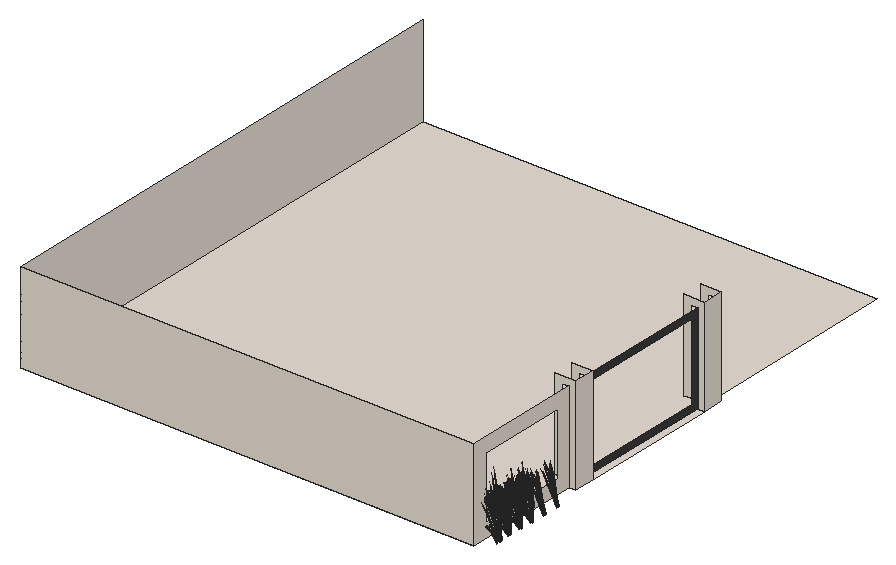
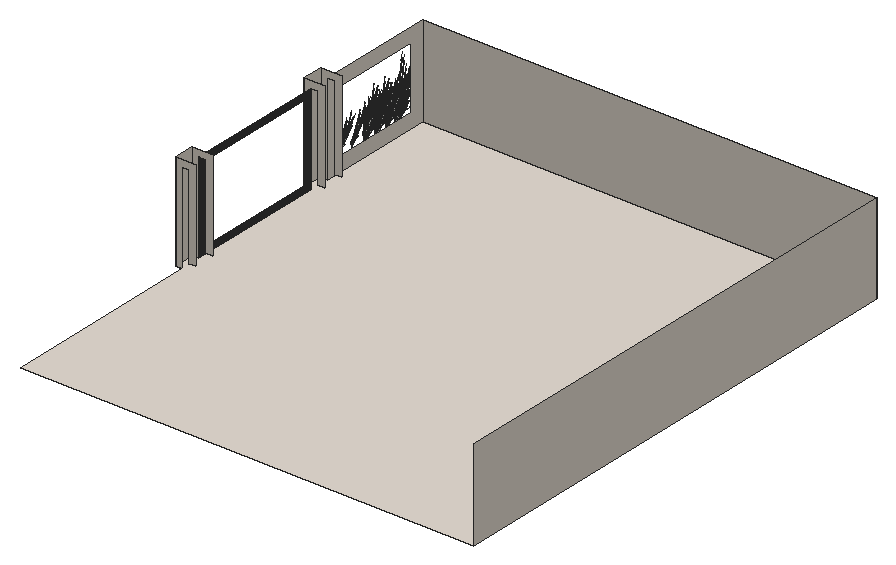
# SketchUp Ruby script. Lengths in inches.
U = 1.inch
M = Sketchup.active_model
def pt(a) = Geom::Point3d.new(a.map { |v| v * U })
def face(e, loops, mat)
  f = e.add_face(loops[0].map { |a| pt(a) })
  loops[1..].each { |l| e.add_face(l.map { |a| pt(a) }).erase! }
  f.material = f.back_material = mat if mat
  f
end
# faces: each face lists its corners as indices into pts; further lists are holes
def faces(e, pts, list, mat = nil) = list.each { |f| face(e, (f[0].is_a?(Array) ? f : [f]).map { |l| l.map { |i| pts[i] } }, mat) }
# xy, xz, yz: faces in a plane at the given z, y or x. An outline is a flat list of corners, or four numbers for a rectangle; further outlines are holes
def ring(l) = l.size == 4 ? [[l[0], l[1]], [l[2], l[1]], [l[2], l[3]], [l[0], l[3]]] : l.each_slice(2).to_a
def flat(e, list, mat, &to3) = list.each { |f| face(e, (f[0].is_a?(Array) ? f : [f]).map { |l| ring(l).map { |u, v| to3.(u, v) } }, mat) }
def xy(e, z, list, mat = nil) = flat(e, list, mat) { |x, y| [x, y, z] }
def xz(e, y, list, mat = nil) = flat(e, list, mat) { |x, z| [x, y, z] }
def yz(e, x, list, mat = nil) = flat(e, list, mat) { |y, z| [x, y, z] }
def lines(e, pts, list) = list.each { |a, b| e.add_line(pt(pts[a]), pt(pts[b])) }
# prism: a flat outline (further loops are holes) pulled along v
def prism(e, loops, v, mat = nil)
  f = face(e, loops, mat); d = Geom::Vector3d.new(v.map { |x| x * U })
  f.pushpull(f.normal.samedirection?(d) ? d.length : -d.length)
end
def box(e, o, s, mat = nil) = prism(e, [[o, [o[0] + s[0], o[1], o[2]], [o[0] + s[0], o[1] + s[1], o[2]], [o[0], o[1] + s[1], o[2]]]], [0, 0, s[2]], mat)
def at(x, y, z, deg = 0) = Geom::Transformation.translation(pt([x, y, z])) * Geom::Transformation.rotation(ORIGIN, Z_AXIS, deg.degrees)
def axes(o, x, y, z) = Geom::Transformation.new([*x, 0, *y, 0, *z, 0, *pt(o).to_a, 1])
def part(name) = M.definitions.add(name)
# library, detail: a bought-in or finely detailed component or shape, given as its bounding box
def library(name, o, s) = part(name).tap { |d| box(d.entities, o, s) }
def detail(e, o, s) = box(e.add_group.entities, o, s)
def put(e, d, t, mat = nil) = e.add_instance(d, t).tap { |i| i.material = mat if mat }
def group(e, t, mat = nil) = e.add_group.tap { |g| g.transformation = t; g.material = mat if mat }.entities
root = M.entities
M.materials.add("LightPink_Translucent").color = [144, 107, 117]
M.materials["LightPink_Translucent"].alpha = 0.75
M.materials.add("M07_Charcoal_Gleam").color = [58, 58, 58]
M.materials.add("Marble_01_1K").color = [230, 221, 211]
c1 = part("blade")
p = [[2.15,0.21,22],[0,0.17,0],[0.09,0.45,0],[2.18,0.31,22],[2.29,0.31,22],[0.38,0.45,0],
  [2.48,0.24,33],[2.49,0.24,33],[2.48,0.22,33]]
faces(c1.entities,p,[[0,1,2,3],[4,5,2,3],[6,3,4,7],[8,0,3,6]])
c2 = part("seeds")
p = [[0.3,-0.1,1.38],[-0.01,-0.03,1.59],[-0.01,-0.03,0.03],[0.14,-0.07,-0.07],[0.29,-0.03,3],[0.15,0.01,3.11]]
faces(c2.entities,p,[[0,1,2,3],[1,0,4,5]],"LightPink_Translucent")
c3 = part("blade with seeds")
put(c3.entities,c1,at(0,0,0))
put(c3.entities,c2,axes([2.4,0.25,30.99],[1.5799,-0.05474,1.17369],[-0.12525,1.92788,0.29478],[-0.07173,-0.02425,1.56792]))
xy(root,-12,[[0,0,0,432,390,432,390,258,396,258,396,240,390,240,390,120,396,120,396,102,390,102,390,0],[390,120,396,240]],"Marble_01_1K")
xz(root,0,[[0,-12,390,66]],"Marble_01_1K")
xz(root,102,[[390,-12,396,-12,396,72,378,72,378,-6,384,-6,384,66,390,66]],"Marble_01_1K")
xz(root,120,[[390,-12,390,66,384,66,384,-6,378,-6,378,72,396,72,396,-12]],"Marble_01_1K")
xz(root,240,[[390,-12,396,-12,396,72,378,72,378,-6,384,-6,384,66,390,66]],"Marble_01_1K")
xz(root,258,[[390,-12,390,66,384,66,384,-6,378,-6,378,72,396,72,396,-12]],"Marble_01_1K")
yz(root,0,[[0,-12,432,66]],"Marble_01_1K")
yz(root,390,[[[120,-12,240,66],[126,-6,234,60]]],"M07_Charcoal_Gleam")
yz(root,390,[[[0,-12,102,66],[12,0,90,54]]],"Marble_01_1K")
yz(root,396,[[102,-12,120,72],[240,-12,258,72]],"Marble_01_1K")
put(root,c3,axes([401.01,11.33,-8.39],[0.21212,-0.01231,1.59586],[-0.14072,0.53355,0.12904],[-0.3023,-0.033,0.68222]))
put(root,c3,axes([401.25,33.91,-8.39],[0.21212,-0.01231,1.59586],[-0.14072,0.53355,0.12904],[-0.3023,-0.033,0.68222]))
put(root,c3,axes([401.28,45.77,-8.39],[0.21212,-0.01231,1.59586],[-0.14072,0.53355,0.12904],[-0.3023,-0.033,0.68222]))
put(root,c3,axes([401.1,12.27,-8.39],[0.17745,-0.11497,1.59586],[0.14939,0.53127,0.12904],[-0.27857,0.12007,0.68222]))
put(root,c3,axes([401.63,21.93,-8.39],[0.21212,-0.01231,1.59586],[-0.14072,0.53355,0.12904],[-0.3023,-0.033,0.68222]))
put(root,c3,axes([400.55,13.17,-9.59],[0.17773,0.04462,1.33163],[0.11455,0.45576,-0.28638],[-0.24142,0.08531,0.56934]))
put(root,c3,axes([401.34,34.85,-8.39],[0.17745,-0.11497,1.59586],[0.14939,0.53127,0.12904],[-0.27857,0.12007,0.68222]))
put(root,c3,axes([401.36,46.71,-8.39],[0.17745,-0.11497,1.59586],[0.14939,0.53127,0.12904],[-0.27857,0.12007,0.68222]))
put(root,c3,axes([402.12,11.71,-8.89],[0.14537,-0.07863,1.64882],[0.05013,0.549,0.12904],[-0.31487,0.07285,0.5893]))
put(root,c3,axes([400.79,35.76,-9.59],[0.17773,0.04462,1.33163],[0.11455,0.45576,-0.28638],[-0.24142,0.08531,0.56934]))
put(root,c3,axes([400.8125,47.62,-9.59],[0.17773,0.04462,1.33163],[0.11455,0.45576,-0.28638],[-0.24142,0.08531,0.56934]))
put(root,c3,axes([402.36,34.3,-8.89],[0.14537,-0.07863,1.64882],[0.05013,0.549,0.12904],[-0.31487,0.07285,0.5893]))
put(root,c3,axes([402.38,46.16,-8.89],[0.14537,-0.07863,1.64882],[0.05013,0.549,0.12904],[-0.31487,0.07285,0.5893]))
put(root,c3,axes([401.72,22.87,-8.39],[0.17745,-0.11497,1.59586],[0.14939,0.53127,0.12904],[-0.27857,0.12007,0.68222]))
put(root,c3,axes([400.56,12.08,-7.61],[-0.08351,0.07057,1.62908],[0.0071,0.51561,-0.25764],[-0.19143,0.06705,0.13065]))
put(root,c3,axes([401.65,10.83,-7.36],[-0.51122,-0.01309,-0.66157],[0.03434,-0.5511,0.07984],[-0.21658,-0.05816,0.93586]))
put(root,c3,axes([401.23,10.97,-9.59],[0.09985,0.15133,1.33163],[-0.23008,0.41134,-0.28638],[-0.23625,-0.09832,0.56934]))
put(root,c3,axes([401.16,23.77,-9.59],[0.17773,0.04462,1.33163],[0.11455,0.45576,-0.28638],[-0.24142,0.08531,0.56934]))
put(root,c3,axes([400.82,11.79,-7.78],[-0.42502,-0.15163,-0.32977],[0.12396,-0.44238,0.42575],[-0.17112,0.04056,0.81462]))
put(root,c3,axes([401.41,10.47,-8.39],[0.18996,0.09365,1.59586],[-0.39312,0.39287,0.12904],[-0.24502,-0.17723,0.68222]))
put(root,c3,axes([400.8,34.67,-7.61],[-0.08351,0.07057,1.62908],[0.0071,0.51561,-0.25764],[-0.19143,0.06705,0.13065]))
put(root,c3,axes([400.82,46.52,-7.61],[-0.08351,0.07057,1.62908],[0.0071,0.51561,-0.25764],[-0.19143,0.06705,0.13065]))
put(root,c3,axes([401.89,33.42,-7.36],[-0.51122,-0.01309,-0.66157],[0.03434,-0.5511,0.07984],[-0.21658,-0.05816,0.93586]))
put(root,c3,axes([402.74,22.3125,-8.89],[0.14537,-0.07863,1.64882],[0.05013,0.549,0.12904],[-0.31487,0.07285,0.5893]))
put(root,c3,axes([401.91,45.28,-7.36],[-0.51122,-0.01309,-0.66157],[0.03434,-0.5511,0.07984],[-0.21658,-0.05816,0.93586]))
put(root,c3,axes([401.48,33.55,-9.59],[0.09985,0.15133,1.33163],[-0.23008,0.41134,-0.28638],[-0.23625,-0.09832,0.56934]))
put(root,c3,axes([401.5,45.41,-9.59],[0.09985,0.15133,1.33163],[-0.23008,0.41134,-0.28638],[-0.23625,-0.09832,0.56934]))
put(root,c3,axes([399.63,12.6,-7.62],[0.06527,0.01458,1.65179],[0.20191,0.48025,-0.15608],[-0.1336,0.12605,0.29231]))
put(root,c3,axes([401.12,12.01,-7.64],[-0.13855,0.49442,-0.47583],[-0.47502,-0.16947,-0.36857],[-0.19125,0.04534,0.91046]))
put(root,c3,axes([401.07,34.37,-7.78],[-0.42502,-0.15163,-0.32977],[0.12396,-0.44238,0.42575],[-0.17112,0.04056,0.81462]))
put(root,c3,axes([401.09,46.23,-7.78],[-0.42502,-0.15163,-0.32977],[0.12396,-0.44238,0.42575],[-0.17112,0.04056,0.81462]))
put(root,c3,axes([401.66,33.06,-8.39],[0.18996,0.09365,1.59586],[-0.39312,0.39287,0.12904],[-0.24502,-0.17723,0.68222]))
put(root,c3,axes([401.68,44.92,-8.39],[0.18996,0.09365,1.59586],[-0.39312,0.39287,0.12904],[-0.24502,-0.17723,0.68222]))
put(root,c3,axes([401.48,10.94,-7.64],[-0.37135,0.36005,-0.47583],[-0.32522,-0.38035,-0.36857],[-0.18868,-0.05478,0.91046]))
put(root,c3,axes([400.875,11.98,-10.61],[0.01297,0.08566,1.6421],[-0.26146,0.44735,-0.25086],[-0.18572,-0.02255,0.2797]))
put(root,c3,axes([399.87,35.1875,-7.62],[0.06527,0.01458,1.65179],[0.20191,0.48025,-0.15608],[-0.1336,0.12605,0.29231]))
put(root,c3,axes([401.17,22.68,-7.61],[-0.08351,0.07057,1.62908],[0.0071,0.51561,-0.25764],[-0.19143,0.06705,0.13065]))
put(root,c3,axes([401.36,34.6,-7.64],[-0.13855,0.49442,-0.47583],[-0.47502,-0.16947,-0.36857],[-0.19125,0.04534,0.91046]))
put(root,c3,axes([399.89,47.05,-7.62],[0.06527,0.01458,1.65179],[0.20191,0.48025,-0.15608],[-0.1336,0.12605,0.29231]))
put(root,c3,axes([402.26,21.43,-7.36],[-0.51122,-0.01309,-0.66157],[0.03434,-0.5511,0.07984],[-0.21658,-0.05816,0.93586]))
put(root,c3,axes([400.95,9.93,-7.62],[0.03791,0.05424,1.65179],[-0.18278,0.48761,-0.15608],[-0.18511,0.00353,0.29231]))
put(root,c3,axes([401.38,46.46,-7.64],[-0.13855,0.49442,-0.47583],[-0.47502,-0.16947,-0.36857],[-0.19125,0.04534,0.91046]))
put(root,c3,axes([401.85,21.56,-9.59],[0.09985,0.15133,1.33163],[-0.23008,0.41134,-0.28638],[-0.23625,-0.09832,0.56934]))
put(root,c3,axes([401.72,33.53,-7.64],[-0.37135,0.36005,-0.47583],[-0.32522,-0.38035,-0.36857],[-0.18868,-0.05478,0.91046]))
put(root,c3,axes([400.18,14.13,-9.42],[0.21313,-0.24635,1.06958],[0.0841,0.38999,0.78586],[-0.15402,0.06983,0.23558]))
put(root,c3,axes([401.74,45.39,-7.64],[-0.37135,0.36005,-0.47583],[-0.32522,-0.38035,-0.36857],[-0.18868,-0.05478,0.91046]))
put(root,c3,axes([401.12,34.57,-10.61],[0.01297,0.08566,1.6421],[-0.26146,0.44735,-0.25086],[-0.18572,-0.02255,0.2797]))
put(root,c3,axes([401.14,46.42,-10.61],[0.01297,0.08566,1.6421],[-0.26146,0.44735,-0.25086],[-0.18572,-0.02255,0.2797]))
put(root,c3,axes([401.44,22.38,-7.78],[-0.42502,-0.15163,-0.32977],[0.12396,-0.44238,0.42575],[-0.17112,0.04056,0.81462]))
put(root,c3,axes([401.375,9.61,-7.61],[-0.11004,-0.00384,1.62908],[-0.35032,0.38367,-0.25764],[-0.18692,-0.07839,0.13065]))
put(root,c3,axes([402.03,21.07,-8.39],[0.18996,0.09365,1.59586],[-0.39312,0.39287,0.12904],[-0.24502,-0.17723,0.68222]))
put(root,c3,axes([400.92,11.73,-7.59],[0.14449,-0.4956,0.447],[0.47502,0.16947,0.36857],[-0.1868,0.02978,0.92496]))
put(root,c3,axes([401.19,32.52,-7.62],[0.03791,0.05424,1.65179],[-0.18278,0.48761,-0.15608],[-0.18511,0.00353,0.29231]))
put(root,c3,axes([401.22,44.38,-7.62],[0.03791,0.05424,1.65179],[-0.18278,0.48761,-0.15608],[-0.18511,0.00353,0.29231]))
put(root,c3,axes([401.09,11.59,-7.3125],[0.25732,0.49218,-0.11324],[-0.45669,0.24187,-0.62851],[-0.19245,0.06494,0.95501]))
put(root,c3,axes([401.67,10.57,-7.3125],[-0.02738,0.55277,-0.11324],[-0.51847,-0.01511,-0.62851],[-0.19968,-0.0384,0.95501]))
put(root,c3,axes([401.34,10.61,-7.78],[-0.29098,-0.34031,-0.32977],[0.33226,-0.32215,0.42575],[-0.16881,-0.04902,0.81462]))
put(root,c3,axes([400.89,11.6,-7.6],[-0.18783,-0.37061,0.05988],[0.34252,-0.1814,0.47138],[-0.15099,0.03579,0.71878]))
put(root,c3,axes([400.42,36.71,-9.42],[0.21313,-0.24635,1.06958],[0.0841,0.38999,0.78586],[-0.15402,0.06983,0.23558]))
put(root,c3,axes([400.25,23.2,-7.62],[0.06527,0.01458,1.65179],[0.20191,0.48025,-0.15608],[-0.1336,0.12605,0.29231]))
put(root,c3,axes([401.73,22.61,-7.64],[-0.13855,0.49442,-0.47583],[-0.47502,-0.16947,-0.36857],[-0.19125,0.04534,0.91046]))
put(root,c3,axes([400.44,48.57,-9.42],[0.21313,-0.24635,1.06958],[0.0841,0.38999,0.78586],[-0.15402,0.06983,0.23558]))
put(root,c3,axes([401.75,12.625,-8.39],[0.12773,-0.16701,1.59586],[0.32252,0.4508,0.12904],[-0.22121,0.20529,0.68222]))
put(root,c3,axes([401.62,32.19,-7.61],[-0.11004,-0.00384,1.62908],[-0.35032,0.38367,-0.25764],[-0.18692,-0.07839,0.13065]))
put(root,c3,axes([400.98,13.0625,-7.78],[-0.44516,0.07768,-0.32977],[-0.11755,-0.44407,0.42575],[-0.12757,0.11927,0.81462]))
put(root,c3,axes([401.64,44.05,-7.61],[-0.11004,-0.00384,1.62908],[-0.35032,0.38367,-0.25764],[-0.18692,-0.07839,0.13065]))
put(root,c3,axes([402.09,21.54,-7.64],[-0.37135,0.36005,-0.47583],[-0.32522,-0.38035,-0.36857],[-0.18868,-0.05478,0.91046]))
put(root,c3,axes([401.17,34.32,-7.59],[0.14449,-0.4956,0.447],[0.47502,0.16947,0.36857],[-0.1868,0.02978,0.92496]))
put(root,c3,axes([401.5,22.58,-10.61],[0.01297,0.08566,1.6421],[-0.26146,0.44735,-0.25086],[-0.18572,-0.02255,0.2797]))
put(root,c3,axes([400.74,14.38,-10.61],[0.0686,0.0543,1.6421],[0.11632,0.50315,-0.25086],[-0.15204,0.10729,0.2797]))
put(root,c3,axes([401.1875,46.17,-7.59],[0.14449,-0.4956,0.447],[0.47502,0.16947,0.36857],[-0.1868,0.02978,0.92496]))
put(root,c3,axes([401.34,34.17,-7.3125],[0.25732,0.49218,-0.11324],[-0.45669,0.24187,-0.62851],[-0.19245,0.06494,0.95501]))
put(root,c3,axes([403.33,72.08,-8.39],[0.21212,-0.01231,1.59586],[-0.14072,0.53355,0.12904],[-0.3023,-0.033,0.68222]))
put(root,c3,axes([403.34,57.84,-8.39],[0.21212,-0.01231,1.59586],[-0.14072,0.53355,0.12904],[-0.3023,-0.033,0.68222]))
put(root,c3,axes([400.64,11.42,-9.42],[0.3265,-0.03889,1.06958],[-0.20711,0.3427,0.78586],[-0.16135,-0.05141,0.23558]))
put(root,c3,axes([401.36,46.03,-7.3125],[0.25732,0.49218,-0.11324],[-0.45669,0.24187,-0.62851],[-0.19245,0.06494,0.95501]))
put(root,c3,axes([401.91,33.15,-7.3125],[-0.02738,0.55277,-0.11324],[-0.51847,-0.01511,-0.62851],[-0.19968,-0.0384,0.95501]))
put(root,c3,axes([401.58,33.19,-7.78],[-0.29098,-0.34031,-0.32977],[0.33226,-0.32215,0.42575],[-0.16881,-0.04902,0.81462]))
put(root,c3,axes([401.9375,45.01,-7.3125],[-0.02738,0.55277,-0.11324],[-0.51847,-0.01511,-0.62851],[-0.19968,-0.0384,0.95501]))
put(root,c3,axes([401.6,45.05,-7.78],[-0.29098,-0.34031,-0.32977],[0.33226,-0.32215,0.42575],[-0.16881,-0.04902,0.81462]))
put(root,c3,axes([401.13,34.18,-7.6],[-0.18783,-0.37061,0.05988],[0.34252,-0.1814,0.47138],[-0.15099,0.03579,0.71878]))
put(root,c3,axes([401.15,46.04,-7.6],[-0.18783,-0.37061,0.05988],[0.34252,-0.1814,0.47138],[-0.15099,0.03579,0.71878]))
put(root,c3,axes([401.57,20.53,-7.62],[0.03791,0.05424,1.65179],[-0.18278,0.48761,-0.15608],[-0.18511,0.00353,0.29231]))
put(root,c3,axes([401.99,35.21,-8.39],[0.12773,-0.16701,1.59586],[0.32252,0.4508,0.12904],[-0.22121,0.20529,0.68222]))
put(root,c3,axes([401.22,35.65,-7.78],[-0.44516,0.07768,-0.32977],[-0.11755,-0.44407,0.42575],[-0.12757,0.11927,0.81462]))
put(root,c3,axes([402.01,47.07,-8.39],[0.12773,-0.16701,1.59586],[0.32252,0.4508,0.12904],[-0.22121,0.20529,0.68222]))
put(root,c3,axes([401.25,47.51,-7.78],[-0.44516,0.07768,-0.32977],[-0.11755,-0.44407,0.42575],[-0.12757,0.11927,0.81462]))
put(root,c3,axes([401.04,12.97,-7.59],[-0.12683,-0.50025,0.447],[0.49754,-0.08682,0.36857],[-0.14663,0.11765,0.92496]))
put(root,c3,axes([400.79,24.73,-9.42],[0.21313,-0.24635,1.06958],[0.0841,0.38999,0.78586],[-0.15402,0.06983,0.23558]))
put(root,c3,axes([400.98,36.97,-10.61],[0.0686,0.0543,1.6421],[0.11632,0.50315,-0.25086],[-0.15204,0.10729,0.2797]))
put(root,c3,axes([401,48.82,-10.61],[0.0686,0.0543,1.6421],[0.11632,0.50315,-0.25086],[-0.15204,0.10729,0.2797]))
put(root,c3,axes([401.99,20.21,-7.61],[-0.11004,-0.00384,1.62908],[-0.35032,0.38367,-0.25764],[-0.18692,-0.07839,0.13065]))
put(root,c3,axes([400.88,34.01,-9.42],[0.3265,-0.03889,1.06958],[-0.20711,0.3427,0.78586],[-0.16135,-0.05141,0.23558]))
put(root,c3,axes([401.29,10.48,-7.26],[0.42234,-0.40113,0.50064],[0.36424,0.42599,0.4128],[-0.19815,-0.07399,1.03595]))
put(root,c3,axes([400.9,45.86,-9.42],[0.3265,-0.03889,1.06958],[-0.20711,0.3427,0.78586],[-0.16135,-0.05141,0.23558]))
put(root,c3,axes([400.9375,12.87,-7.6],[-0.35109,-0.22859,0.05988],[0.2044,-0.32553,0.47138],[-0.11256,0.10524,0.71878]))
put(root,c3,axes([401.54,22.33,-7.59],[0.14449,-0.4956,0.447],[0.47502,0.16947,0.36857],[-0.1868,0.02978,0.92496]))
put(root,c3,axes([401.71,22.1875,-7.3125],[0.25732,0.49218,-0.11324],[-0.45669,0.24187,-0.62851],[-0.19245,0.06494,0.95501]))
put(root,c3,axes([402.29,21.16,-7.3125],[-0.02738,0.55277,-0.11324],[-0.51847,-0.01511,-0.62851],[-0.19968,-0.0384,0.95501]))
put(root,c3,axes([401.28,35.55,-7.59],[-0.12683,-0.50025,0.447],[0.49754,-0.08682,0.36857],[-0.14663,0.11765,0.92496]))
put(root,c3,axes([401.96,21.2,-7.78],[-0.29098,-0.34031,-0.32977],[0.33226,-0.32215,0.42575],[-0.16881,-0.04902,0.81462]))
put(root,c3,axes([401.3,47.41,-7.59],[-0.12683,-0.50025,0.447],[0.49754,-0.08682,0.36857],[-0.14663,0.11765,0.92496]))
put(root,c3,axes([401.51,22.2,-7.6],[-0.18783,-0.37061,0.05988],[0.34252,-0.1814,0.47138],[-0.15099,0.03579,0.71878]))
put(root,c3,axes([401.65,13.04,-8.39],[0.09522,-0.18683,1.59586],[0.39947,0.38663,0.12904],[-0.18021,0.24097,0.68222]))
put(root,c3,axes([402.37,23.22,-8.39],[0.12773,-0.16701,1.59586],[0.32252,0.4508,0.12904],[-0.22121,0.20529,0.68222]))
put(root,c3,axes([401.6,23.66,-7.78],[-0.44516,0.07768,-0.32977],[-0.11755,-0.44407,0.42575],[-0.12757,0.11927,0.81462]))
put(root,c3,axes([401.54,33.0625,-7.26],[0.42234,-0.40113,0.50064],[0.36424,0.42599,0.4128],[-0.19815,-0.07399,1.03595]))
put(root,c3,axes([401.56,44.92,-7.26],[0.42234,-0.40113,0.50064],[0.36424,0.42599,0.4128],[-0.19815,-0.07399,1.03595]))
put(root,c3,axes([403.42,73.02,-8.39],[0.17745,-0.11497,1.59586],[0.14939,0.53127,0.12904],[-0.27857,0.12007,0.68222]))
put(root,c3,axes([403.43,58.78,-8.39],[0.17745,-0.11497,1.59586],[0.14939,0.53127,0.12904],[-0.27857,0.12007,0.68222]))
put(root,c3,axes([401.18,35.45,-7.6],[-0.35109,-0.22859,0.05988],[0.2044,-0.32553,0.47138],[-0.11256,0.10524,0.71878]))
put(root,c3,axes([401.2,47.3125,-7.6],[-0.35109,-0.22859,0.05988],[0.2044,-0.32553,0.47138],[-0.11256,0.10524,0.71878]))
put(root,c3,axes([401.36,24.98,-10.61],[0.0686,0.0543,1.6421],[0.11632,0.50315,-0.25086],[-0.15204,0.10729,0.2797]))
put(root,c3,axes([401.27,11.74,-7.3],[0.42502,0.15163,0.32977],[-0.12396,0.44238,-0.42575],[-0.17112,0.04056,0.81462]))
put(root,c3,axes([401.26,22.02,-9.42],[0.3265,-0.03889,1.06958],[-0.20711,0.3427,0.78586],[-0.16135,-0.05141,0.23558]))
put(root,c3,axes([402.87,73.93,-9.59],[0.17773,0.04462,1.33163],[0.11455,0.45576,-0.28638],[-0.24142,0.08531,0.56934]))
put(root,c3,axes([402.875,59.69,-9.59],[0.17773,0.04462,1.33163],[0.11455,0.45576,-0.28638],[-0.24142,0.08531,0.56934]))
put(root,c3,axes([401.35,13.11,-7.64],[0.13138,0.49631,-0.47583],[-0.49754,0.08682,-0.36857],[-0.14258,0.13331,0.91046]))
put(root,c3,axes([401.9,35.62,-8.39],[0.09522,-0.18683,1.59586],[0.39947,0.38663,0.12904],[-0.18021,0.24097,0.68222]))
put(root,c3,axes([401.92,47.48,-8.39],[0.09522,-0.18683,1.59586],[0.39947,0.38663,0.12904],[-0.18021,0.24097,0.68222]))
put(root,c3,axes([401.49,10.47,-7.6],[0.02575,-0.41332,0.05988],[0.38885,0.01133,0.47138],[-0.14895,-0.04325,0.71878]))
put(root,c3,axes([400.57,14.01,-7.61],[-0.01271,0.10756,1.62908],[0.36076,0.37419,-0.25764],[-0.09444,0.17695,0.13065]))
put(root,c3,axes([401.66,23.5625,-7.59],[-0.12683,-0.50025,0.447],[0.49754,-0.08682,0.36857],[-0.14663,0.11765,0.92496]))
put(root,c3,axes([404.44,72.47,-8.89],[0.14537,-0.07863,1.64882],[0.05013,0.549,0.12904],[-0.31487,0.07285,0.5893]))
put(root,c3,axes([404.45,58.23,-8.89],[0.14537,-0.07863,1.64882],[0.05013,0.549,0.12904],[-0.31487,0.07285,0.5893]))
put(root,c3,axes([402.59,12.76,-10.08],[-0.53199,-0.08911,-0.58063],[0.11226,-0.54969,-0.15239],[-0.15876,-0.06661,1.28164]))
put(root,c3,axes([402.68,9.76,-6.94],[-0.34131,0.52108,-0.12682],[-0.49429,-0.3002,-0.70393],[-0.17182,-0.14722,1.06961]))
put(root,c3,axes([401.52,34.32,-7.3],[0.42502,0.15163,0.32977],[-0.12396,0.44238,-0.42575],[-0.17112,0.04056,0.81462]))
put(root,c3,axes([401.91,21.08,-7.26],[0.42234,-0.40113,0.50064],[0.36424,0.42599,0.4128],[-0.19815,-0.07399,1.03595]))
put(root,c3,axes([401.54,46.18,-7.3],[0.42502,0.15163,0.32977],[-0.12396,0.44238,-0.42575],[-0.17112,0.04056,0.81462]))
put(root,c3,axes([401.75,10.78,-7.3],[0.29098,0.34031,0.32977],[-0.33226,0.32215,-0.42575],[-0.16881,-0.04902,0.81462]))
put(root,c3,axes([401.56,23.47,-7.6],[-0.35109,-0.22859,0.05988],[0.2044,-0.32553,0.47138],[-0.11256,0.10524,0.71878]))
put(root,c3,axes([401.59,35.7,-7.64],[0.13138,0.49631,-0.47583],[-0.49754,0.08682,-0.36857],[-0.14258,0.13331,0.91046]))
put(root,c3,axes([402.53,10.18,-7.36],[-0.43608,-0.26272,-0.66157],[0.30991,-0.46038,0.07984],[-0.158,-0.15687,0.93586]))
put(root,c3,axes([401.61,47.56,-7.64],[0.13138,0.49631,-0.47583],[-0.49754,0.08682,-0.36857],[-0.14258,0.13331,0.91046]))
put(root,c3,axes([402.33,10.2,-7.64],[-0.50465,0.12921,-0.47583],[-0.08828,-0.48932,-0.36857],[-0.13555,-0.14022,0.91046]))
put(root,c3,axes([401.73,33.06,-7.6],[0.02575,-0.41332,0.05988],[0.38885,0.01133,0.47138],[-0.14895,-0.04325,0.71878]))
put(root,c3,axes([400.8125,36.59,-7.61],[-0.01271,0.10756,1.62908],[0.36076,0.37419,-0.25764],[-0.09444,0.17695,0.13065]))
put(root,c3,axes([401.75,44.92,-7.6],[0.02575,-0.41332,0.05988],[0.38885,0.01133,0.47138],[-0.14895,-0.04325,0.71878]))
put(root,c3,axes([400.84,48.45,-7.61],[-0.01271,0.10756,1.62908],[0.36076,0.37419,-0.25764],[-0.09444,0.17695,0.13065]))
put(root,c3,axes([402.83,35.34,-10.08],[-0.53199,-0.08911,-0.58063],[0.11226,-0.54969,-0.15239],[-0.15876,-0.06661,1.28164]))
put(root,c3,axes([402.93,32.34,-6.94],[-0.34131,0.52108,-0.12682],[-0.49429,-0.3002,-0.70393],[-0.17182,-0.14722,1.06961]))
put(root,c3,axes([402.27,23.63,-8.39],[0.09522,-0.18683,1.59586],[0.39947,0.38663,0.12904],[-0.18021,0.24097,0.68222]))
put(root,c3,axes([402.85,47.2,-10.08],[-0.53199,-0.08911,-0.58063],[0.11226,-0.54969,-0.15239],[-0.15876,-0.06661,1.28164]))
put(root,c3,axes([402.95,44.2,-6.94],[-0.34131,0.52108,-0.12682],[-0.49429,-0.3002,-0.70393],[-0.17182,-0.14722,1.06961]))
put(root,c3,axes([401.89,13.8,-10.12],[-0.47863,-0.27177,-0.46235],[0.28609,-0.48733,0],[-0.10901,-0.0619,1.46668]))
put(root,c3,axes([401.99,33.37,-7.3],[0.29098,0.34031,0.32977],[-0.33226,0.32215,-0.42575],[-0.16881,-0.04902,0.81462]))
put(root,c3,axes([402.88,72.84,-7.61],[-0.08351,0.07057,1.62908],[0.0071,0.51561,-0.25764],[-0.19143,0.06705,0.13065]))
put(root,c3,axes([402.89,58.59,-7.61],[-0.08351,0.07057,1.62908],[0.0071,0.51561,-0.25764],[-0.19143,0.06705,0.13065]))
put(root,c3,axes([402.02,45.23,-7.3],[0.29098,0.34031,0.32977],[-0.33226,0.32215,-0.42575],[-0.16881,-0.04902,0.81462]))
put(root,c3,axes([401.68,9.75,-10.61],[-0.04954,0.0716,1.6421],[-0.50062,0.15438,-0.25086],[-0.12094,-0.14044,0.2797]))
put(root,c3,axes([403.97,71.59,-7.36],[-0.51122,-0.01309,-0.66157],[0.03434,-0.5511,0.07984],[-0.21658,-0.05816,0.93586]))
put(root,c3,axes([401.11,12.76,-7.3125],[0.47307,0.29971,-0.11324],[-0.27254,0.43404,-0.62851],[-0.13365,0.15087,0.95501]))
put(root,c3,axes([403.97,57.35,-7.36],[-0.51122,-0.01309,-0.66157],[0.03434,-0.5511,0.07984],[-0.21658,-0.05816,0.93586]))
put(root,c3,axes([402.78,32.77,-7.36],[-0.43608,-0.26272,-0.66157],[0.30991,-0.46038,0.07984],[-0.158,-0.15687,0.93586]))
put(root,c3,axes([402.57,32.78,-7.64],[-0.50465,0.12921,-0.47583],[-0.08828,-0.48932,-0.36857],[-0.13555,-0.14022,0.91046]))
put(root,c3,axes([402.8,44.625,-7.36],[-0.43608,-0.26272,-0.66157],[0.30991,-0.46038,0.07984],[-0.158,-0.15687,0.93586]))
put(root,c3,axes([403.56,71.72,-9.59],[0.09985,0.15133,1.33163],[-0.23008,0.41134,-0.28638],[-0.23625,-0.09832,0.56934]))
put(root,c3,axes([401.89,22.34,-7.3],[0.42502,0.15163,0.32977],[-0.12396,0.44238,-0.42575],[-0.17112,0.04056,0.81462]))
put(root,c3,axes([403.5625,57.48,-9.59],[0.09985,0.15133,1.33163],[-0.23008,0.41134,-0.28638],[-0.23625,-0.09832,0.56934]))
put(root,c3,axes([402.6,44.64,-7.64],[-0.50465,0.12921,-0.47583],[-0.08828,-0.48932,-0.36857],[-0.13555,-0.14022,0.91046]))
put(root,c3,axes([402.18,14.125,-9.79],[-0.31974,0.54466,0],[-0.53494,-0.30375,-0.48057],[-0.12184,-0.06918,1.52448]))
put(root,c3,axes([403.15,72.54,-7.78],[-0.42502,-0.15163,-0.32977],[0.12396,-0.44238,0.42575],[-0.17112,0.04056,0.81462]))
put(root,c3,axes([403.15,58.3,-7.78],[-0.42502,-0.15163,-0.32977],[0.12396,-0.44238,0.42575],[-0.17112,0.04056,0.81462]))
put(root,c3,axes([401.97,23.71,-7.64],[0.13138,0.49631,-0.47583],[-0.49754,0.08682,-0.36857],[-0.14258,0.13331,0.91046]))
put(root,c3,axes([403.73,71.23,-8.39],[0.18996,0.09365,1.59586],[-0.39312,0.39287,0.12904],[-0.24502,-0.17723,0.68222]))
put(root,c3,axes([403.74,56.98,-8.39],[0.18996,0.09365,1.59586],[-0.39312,0.39287,0.12904],[-0.24502,-0.17723,0.68222]))
